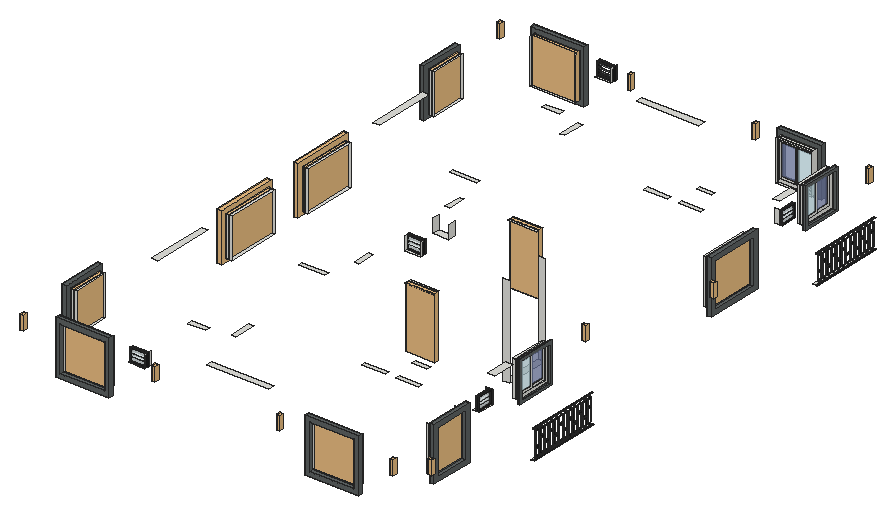
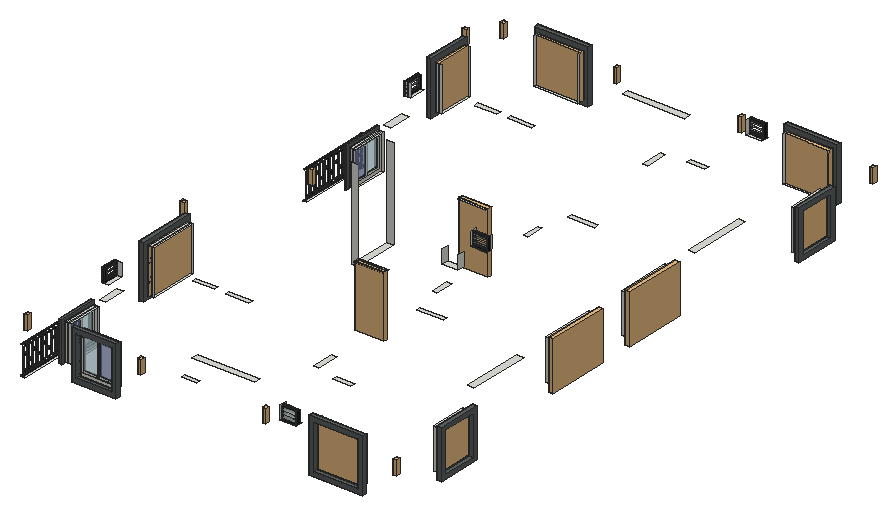
# SketchUp Ruby script. Lengths in inches.
U = 1.inch
M = Sketchup.active_model
def pt(a) = Geom::Point3d.new(a.map { |v| v * U })
def face(e, loops, mat)
  f = e.add_face(loops[0].map { |a| pt(a) })
  loops[1..].each { |l| e.add_face(l.map { |a| pt(a) }).erase! }
  f.material = f.back_material = mat if mat
  f
end
# faces: each face lists its corners as indices into pts; further lists are holes
def faces(e, pts, list, mat = nil) = list.each { |f| face(e, (f[0].is_a?(Array) ? f : [f]).map { |l| l.map { |i| pts[i] } }, mat) }
# xy, xz, yz: faces in a plane at the given z, y or x. An outline is a flat list of corners, or four numbers for a rectangle; further outlines are holes
def ring(l) = l.size == 4 ? [[l[0], l[1]], [l[2], l[1]], [l[2], l[3]], [l[0], l[3]]] : l.each_slice(2).to_a
def flat(e, list, mat, &to3) = list.each { |f| face(e, (f[0].is_a?(Array) ? f : [f]).map { |l| ring(l).map { |u, v| to3.(u, v) } }, mat) }
def xy(e, z, list, mat = nil) = flat(e, list, mat) { |x, y| [x, y, z] }
def xz(e, y, list, mat = nil) = flat(e, list, mat) { |x, z| [x, y, z] }
def yz(e, x, list, mat = nil) = flat(e, list, mat) { |y, z| [x, y, z] }
def lines(e, pts, list) = list.each { |a, b| e.add_line(pt(pts[a]), pt(pts[b])) }
# prism: a flat outline (further loops are holes) pulled along v
def prism(e, loops, v, mat = nil)
  f = face(e, loops, mat); d = Geom::Vector3d.new(v.map { |x| x * U })
  f.pushpull(f.normal.samedirection?(d) ? d.length : -d.length)
end
def box(e, o, s, mat = nil) = prism(e, [[o, [o[0] + s[0], o[1], o[2]], [o[0] + s[0], o[1] + s[1], o[2]], [o[0], o[1] + s[1], o[2]]]], [0, 0, s[2]], mat)
def at(x, y, z, deg = 0) = Geom::Transformation.translation(pt([x, y, z])) * Geom::Transformation.rotation(ORIGIN, Z_AXIS, deg.degrees)
def axes(o, x, y, z) = Geom::Transformation.new([*x, 0, *y, 0, *z, 0, *pt(o).to_a, 1])
def part(name) = M.definitions.add(name)
# library, detail: a bought-in or finely detailed component or shape, given as its bounding box
def library(name, o, s) = part(name).tap { |d| box(d.entities, o, s) }
def detail(e, o, s) = box(e.add_group.entities, o, s)
def put(e, d, t, mat = nil) = e.add_instance(d, t).tap { |i| i.material = mat if mat }
def group(e, t, mat = nil) = e.add_group.tap { |g| g.transformation = t; g.material = mat if mat }.entities
root = M.entities
M.materials.add("1487 AP 8286 CHARCOAL SHADOW").color = [94, 99, 99]
M.materials.add("[Color M08]").color = [30, 30, 30]
M.materials.add("[Color_008]1").color = [30, 30, 30]
M.materials.add("[Translucent Glass Safety]").color = [218, 227, 229]
M.materials["[Translucent Glass Safety]"].alpha = 0.5
M.materials.add("[Translucent_Glass_Safety]").color = [204, 235, 244]
M.materials["[Translucent_Glass_Safety]"].alpha = 0.5
M.materials.add("[Translucent_Glass_Sky_Reflection]").color = [125, 138, 183]
M.materials["[Translucent_Glass_Sky_Reflection]"].alpha = 0.52
c1 = library("porta 4",[0.2,-5.42,1.33],[46.55,4.72,83.21])
c2 = part("Group\#70")
prism(c2.entities,[[[4.13,0,3.9375],[7.875,0,3.9375],[7.875,0,13.78],[4.13,0,13.78],[4.13,0,15.75],[7.875,0,15.75],[7.875,0,35.43],[4.13,0,35.43],[4.13,0,39.37],[3.74,0,39.37],[3.74,0,35.43],[0,0,35.43],[0,0,15.75],[3.74,0,15.75],[3.74,0,13.78],[0,0,13.78],[0,0,3.9375],[3.74,0,3.9375],[3.74,0,0],[4.13,0,0]],[[0.39,0,16.14],[0.39,0,35.04],[7.48,0,35.04],[7.48,0,16.14]],[[7.48,0,4.33],[0.39,0,4.33],[0.39,0,13.39],[7.48,0,13.39]]],[0,0.39,0],"[Color M08]")
c3 = part("Group\#69")
prism(c3.entities,[[[3.74,0,35.43],[0,0,35.43],[0,0,25.59],[3.74,0,25.59],[3.74,0,23.62],[0,0,23.62],[0,0,3.9375],[3.74,0,3.9375],[3.74,0,0],[4.13,0,0],[4.13,0,3.9375],[7.875,0,3.9375],[7.875,0,23.62],[4.13,0,23.62],[4.13,0,25.59],[7.875,0,25.59],[7.875,0,35.43],[4.13,0,35.43],[4.13,0,39.37],[3.74,0,39.37]],[[7.48,0,23.23],[7.48,0,4.33],[0.39,0,4.33],[0.39,0,23.23]],[[0.39,0,35.04],[7.48,0,35.04],[7.48,0,25.98],[0.39,0,25.98]]],[0,0.39,0],"[Color M08]")
c4 = part("Group\#71")
put(c4.entities,c2,at(0,0,0))
put(c4.entities,c3,at(9.84,0,0))
c5 = part("Group\#79")
g1 = group(c5.entities,at(0,0,0))
box(g1,[0,-2.09,0],[1.97,122.29,0.79],"[Color M08]")
put(c5.entities,c4,axes([0.79,40.35,0.79],[0,1,0],[1,0,0],[0,0,1]))
put(c5.entities,c4,axes([0.79,79.72,0.79],[0,1,0],[1,0,0],[0,0,1]))
put(c5.entities,c4,axes([0.79,60.04,0.79],[0,1,0],[1,0,0],[0,0,1]))
put(c5.entities,c4,axes([0.79,99.41,0.79],[0,1,0],[1,0,0],[0,0,1]))
g2 = group(c5.entities,at(0,0,40.16))
box(g2,[0,-2.09,0],[1.97,122.29,0.79],"[Color M08]")
put(c5.entities,c4,axes([0.79,20.67,0.79],[0,1,0],[1,0,0],[0,0,1]))
put(c5.entities,c4,axes([0.79,0.98,0.79],[0,1,0],[1,0,0],[0,0,1]))
c6 = part("14")
prism(c6.entities,[[[0,60,66],[0,0,66],[0,0,0],[0,60,0]],[[0,54,6],[0,6,6],[0,6,60],[0,54,60]]],[-6,0,0])
c7 = library("15",[-6,0,0],[6,84,66])
c8 = part("17")
prism(c8.entities,[[[0,0,0],[0,0,72],[72,0,72],[72,0,0]],[[6,0,6],[66,0,6],[66,0,66],[6,0,66]]],[0,-6,0])
c9 = library("Group\#98",[0,-5.45,0],[91.05,108.7,8])
c10 = part("Two-panel window")
xy(c10.entities,0,[[0,0,4.33,55.51]])
xy(c10.entities,2.76,[[0,2.76,2,2.76,2,27.76,0.82,27.76,0.82,52.76,0,52.76],[3.15,2.76,4.33,2.76,4.33,52.76,2.36,52.76,2.36,27.76,3.15,27.76],[0.82,27.76,2.36,52.76]])
xy(c10.entities,4.72,[[2,4.72,2.4,26.38],[2.76,4.72,3.15,26.38],[0.82,29.13,1.22,50.79],[1.97,29.13,2.36,50.79]])
xy(c10.entities,36.61,[[2,4.72,2.4,26.38],[2.76,4.72,3.15,26.38],[0.82,29.13,1.22,50.79],[1.97,29.13,2.36,50.79]])
xy(c10.entities,38.58,[[0,2.76,2,27.76],[3.15,2.76,4.33,27.76],[0,27.76,0.82,52.76],[0.82,27.76,2.36,52.76],[2.36,27.76,4.33,52.76]])
xy(c10.entities,41.34,[[0,0,4.33,55.51]])
xz(c10.entities,0,[[0,0,4.33,41.34]])
xz(c10.entities,2.76,[[0,2.76,2,38.58],[3.15,2.76,4.33,38.58]])
xz(c10.entities,4.72,[[2,4.72,2.4,36.61],[2.76,4.72,3.15,36.61]])
xz(c10.entities,26.38,[[2,4.72,2.4,36.61],[2.76,4.72,3.15,36.61]])
xz(c10.entities,27.76,[[0.82,2.76,2,38.58],[2,2.76,2.36,38.58],[2.36,2.76,3.15,38.58]])
xz(c10.entities,29.13,[[0.82,4.72,1.22,36.61],[1.97,4.72,2.36,36.61]])
xz(c10.entities,50.79,[[0.82,4.72,1.22,36.61],[1.97,4.72,2.36,36.61]])
xz(c10.entities,52.76,[[0,2.76,0.82,38.58],[0.82,2.76,2.36,38.58],[2.36,2.76,4.33,38.58]])
xz(c10.entities,55.51,[[0,0,4.33,41.34]])
yz(c10.entities,0,[[[0,0,55.51,41.34],[2.76,2.76,52.76,38.58]]])
yz(c10.entities,0.82,[[[27.76,2.76,52.76,38.58],[29.13,4.72,50.79,36.61]]])
yz(c10.entities,1.22,[[29.13,4.72,50.79,36.61]],"[Translucent_Glass_Sky_Reflection]")
yz(c10.entities,1.97,[[29.13,4.72,50.79,36.61]],"[Translucent_Glass_Sky_Reflection]")
yz(c10.entities,2,[[[2.76,2.76,27.76,38.58],[4.72,4.72,26.38,36.61]]])
yz(c10.entities,2.36,[[[27.76,2.76,52.76,38.58],[29.13,4.72,50.79,36.61]]])
yz(c10.entities,2.4,[[4.72,4.72,26.38,36.61]],"[Translucent_Glass_Safety]")
yz(c10.entities,2.76,[[4.72,4.72,26.38,36.61]],"[Translucent_Glass_Safety]")
yz(c10.entities,3.15,[[[2.76,2.76,27.76,38.58],[4.72,4.72,26.38,36.61]]])
yz(c10.entities,4.33,[[[0,0,55.51,41.34],[2.76,2.76,52.76,38.58]]])
c11 = library("Group\#36",[0,-5.45,0],[91.05,108.7,8])
c12 = library("Group\#50",[0,-5.45,0],[91.05,108.7,8])
c13 = library("Group\#28",[0.125,0,-2.28],[4,104,84.28])
c14 = library("WALL LIGHT 69",[4.19,4.05,-9.73],[4.61,5.7,19.03])
c15 = part("Group\#40")
box(c15.entities,[0,0.25,0],[21,0.25,6],"[Translucent Glass Safety]")
c16 = part("tingkap keping toilet")
g3 = group(c16.entities,at(-23.5,-2,0),"[Color_008]1")
prism(g3,[[[47,0,57],[22.5,0,57],[22.5,0,41.8],[47,0,41.8]],[[24.5,0,43.3],[24.5,0,55.5],[45.5,0,55.5],[45.5,0,43.3]]],[0,4,0])
g4 = group(c16.entities,at(1,-2,47))
put(g4,c15,axes([0,3.73,3.53],[1,0,0],[0,0.757,0.65342],[0,-0.65342,0.757]))
put(g4,c15,axes([0,3.73,-0.17],[1,0,0],[0,0.757,0.65342],[0,-0.65342,0.757]))
put(g4,c15,axes([0,3.73,-3.87],[1,0,0],[0,0.757,0.65342],[0,-0.65342,0.757]))
xy(root,134,[[682.5,564.97,688.5,663.97],[553.5,678.97,562.5,738.97],[679.5,1044.97,685.5,1143.97]])
xy(root,162,[[649.5,897.97,658.5,963.97]])
xy(root,168,[[218,357.97,278,366.97],[554.5,357.97,614.5,366.97],[171,426.87,180,474.87],[652.5,426.87,661.5,474.87],[493.5,600.97,513.5,606.97],
  [622.5,609.97,631.5,657.97],[198,654.97,207,726.97],[198,783.97,207,855.97],[171,1029.97,180,1077.97],[493.5,1080.97,513.5,1086.97],
  [622.5,1089.97,631.5,1137.97],[218,1143.97,278,1152.97],[550.5,1143.97,598.5,1152.97]])
xy(root,210,[[306,357.97,327.5,366.97],[652.5,504.97,661.5,526.53],[382.75,726.97,404.25,735.97],[382.75,774.97,404.25,783.97],[649.5,1017.47,658.5,1038.97],
  [306,1143.97,327.5,1152.97]])
xy(root,216,[[309,453.97,333,459.97],[360,462.97,366,492.97],[507,498.97,539,504.97],[553.5,498.97,583.5,504.97],[622.5,567.97,631.5,597.97],
  [622.5,609.97,631.5,657.97],[321,624.97,357,630.97],[433.5,663.97,472.5,672.97],[363,666.97,369,690.97],[363,819.97,369,843.97],
  [433.5,837.97,472.5,846.97],[321,879.97,357,885.97],[504,978.97,536,984.97],[550.5,978.97,580.5,984.97],[360,1017.47,366,1047.47],
  [622.5,1047.97,631.5,1077.97],[309,1050.97,333,1056.97],[622.5,1089.97,631.5,1137.97]])
xy(root,222,[[386.25,387.97,470.25,396.97],[171,426.87,180,474.87],[198,530.97,207,614.97],[198,654.97,207,726.97],[198,783.97,207,855.97],
  [649.5,897.97,658.5,963.97],[198,903.97,207,987.97],[171,1029.97,180,1077.97],[386.25,1113.97,470.25,1122.97],[550.5,1143.97,598.5,1152.97]])
xz(root,426.87,[[171,168,180,222],[652.5,168,661.5,228]])
xz(root,474.87,[[171,168,180,222],[652.5,168,661.5,228]])
xz(root,526.53,[[652.5,210,661.5,228]])
xz(root,609.97,[[622.5,168,631.5,216]])
xz(root,654.97,[[198,168,207,222]])
xz(root,657.97,[[622.5,168,631.5,216]])
xz(root,678.97,[[553.5,134,562.5,258]])
xz(root,726.97,[[198,168,207,222]])
xz(root,738.97,[[553.5,134,562.5,258]])
xz(root,783.97,[[198,168,207,222]])
xz(root,855.97,[[198,168,207,222]])
xz(root,897.97,[[649.5,162,658.5,222]])
xz(root,963.97,[[649.5,162,658.5,222]])
xz(root,1017.47,[[649.5,210,658.5,228]])
xz(root,1029.97,[[171,168,180,222]])
xz(root,1077.97,[[171,168,180,222]])
xz(root,1089.97,[[622.5,168,631.5,216]])
xz(root,1137.97,[[622.5,168,631.5,216]])
yz(root,218,[[357.97,168,366.97,228],[1143.97,168,1152.97,228]])
yz(root,278,[[357.97,168,366.97,228],[1143.97,168,1152.97,228]])
yz(root,327.5,[[357.97,210,366.97,228],[1143.97,210,1152.97,228]])
yz(root,382.75,[[726.97,210,735.97,228],[774.97,210,783.97,228]])
yz(root,404.25,[[726.97,210,735.97,228],[774.97,210,783.97,228]])
yz(root,550.5,[[1143.97,168,1152.97,222]])
yz(root,554.5,[[357.97,168,366.97,228]])
yz(root,598.5,[[1143.97,168,1152.97,222]])
yz(root,614.5,[[357.97,168,366.97,228]])
put(root,c1,axes([472.67,670.54,132],[-0.83352,0,0],[0,1,0],[0,0,1]))
put(root,c1,axes([472.67,840.41,132],[-0.83352,0,0],[0,-1,0],[0,0,1]))
put(root,c5,axes([687.5,566.66,134],[-1,0,0],[0,0.80958,0],[0,0,0.9525]))
put(root,c5,axes([684.5,1046.66,134],[-1,0,0],[0,0.80958,0],[0,0,0.9525]))
g5 = group(root,at(658.5,891.97,156),"1487 AP 8286 CHARCOAL SHADOW")
prism(g5,[[[0,0,72],[0,78,72],[0,78,0],[0,0,0]],[[0,6,6],[0,72,6],[0,72,66],[0,6,66]]],[6,0,0])
put(root,c6,at(171,1023.97,162),"1487 AP 8286 CHARCOAL SHADOW")
put(root,c6,at(171,420.87,162),"1487 AP 8286 CHARCOAL SHADOW")
put(root,c7,at(198,777.97,162),"1487 AP 8286 CHARCOAL SHADOW")
put(root,c7,at(198,648.97,162),"1487 AP 8286 CHARCOAL SHADOW")
put(root,c8,at(212,357.97,162),"1487 AP 8286 CHARCOAL SHADOW")
put(root,c8,at(548.5,357.97,162),"1487 AP 8286 CHARCOAL SHADOW")
g6 = group(root,at(661.5,420.87,162),"1487 AP 8286 CHARCOAL SHADOW")
prism(g6,[[[0,0,0],[0,0,72],[0,60,72],[0,60,0]],[[0,6,66],[0,6,6],[0,54,6],[0,54,66]]],[6,0,0])
g7 = group(root,at(544.5,1152.97,162),"1487 AP 8286 CHARCOAL SHADOW")
prism(g7,[[[60,0,66],[0,0,66],[0,0,0],[60,0,0]],[[54,0,6],[6,0,6],[6,0,60],[54,0,60]]],[0,6,0])
g8 = group(root,at(212,1152.97,162),"1487 AP 8286 CHARCOAL SHADOW")
prism(g8,[[[0,0,72],[0,0,0],[72,0,0],[72,0,72]],[[66,0,66],[66,0,6],[6,0,6],[6,0,66]]],[0,6,0])
put(root,c9,axes([652.6,963.97,165.01],[0,-0.72488,0],[0,0,0.55196],[0.55,0,0]))
g9 = group(root,at(631.5,604.97,163),"1487 AP 8286 CHARCOAL SHADOW")
prism(g9,[[[0,56,2],[0,2,2],[0,2,56],[0,56,56]],[[0,53,5],[0,53,53],[0,5,53],[0,5,5]]],[3,0,0])
g10 = group(root,at(631.5,1084.97,163),"1487 AP 8286 CHARCOAL SHADOW")
prism(g10,[[[0,56,2],[0,2,2],[0,2,56],[0,56,56]],[[0,53,5],[0,53,53],[0,5,53],[0,5,5]]],[5,0,0])
put(root,c9,axes([655.6,474.87,171.01],[0,-0.52718,0],[0,0,0.55196],[0.55,0,0]))
put(root,c10,axes([625.67,609.97,168],[1,0,0],[0,0.86468,0],[0,0,1.16114]))
put(root,c10,axes([625.67,1089.97,168],[1,0,0],[0,0.86468,0],[0,0,1.16114]))
put(root,c10,axes([598.5,1147.14,168],[0,1,0],[-0.86468,0,0],[0,0,1.30629]))
put(root,c9,axes([218,363.875,171.01],[0.65898,0,0],[0,0,0.55196],[0,-0.55,0]))
put(root,c11,axes([218,1147.07,171.01],[0.65898,0,0],[0,0,0.55196],[0,0.55,0]))
put(root,c12,axes([554.5,363.875,171.01],[0.65898,0,0],[0,0,0.55196],[0,-0.55,0]))
put(root,c13,axes([198.875,654.97,169.46],[1,0,0],[0,0.69231,0],[0,0,0.64074]))
put(root,c13,axes([198.875,855.97,169.46],[1,0,0],[0,-0.69231,0],[0,0,0.64074]))
put(root,c9,axes([176.9,474.87,170.71],[0,-0.52718,0],[0,0,0.49676],[-0.55,0,0]))
put(root,c9,axes([176.9,1029.97,170.71],[0,0.52718,0],[0,0,0.49676],[-0.55,0,0]))
put(root,c14,at(642,709.2,205.375,90))
put(root,c14,at(699.24,377.55,208.64,90))
put(root,c14,at(696.49,856.8,211.25,90))
put(root,c14,at(505.9375,347.23,212.67))
put(root,c14,axes([173.78,346.73,212.67],[-1,0,0],[0,1,0],[0,0,1]))
put(root,c14,axes([350.5625,347.23,212.67],[-1,0,0],[0,1,0],[0,0,1]))
put(root,c14,at(658.9375,347.23,212.67))
put(root,c14,axes([505.9375,1163.72,212.67],[1,0,0],[0,-1,0],[0,0,1]))
put(root,c14,at(173.78,1164.22,212.67,180))
put(root,c14,at(350.5625,1163.72,212.67,180))
put(root,c14,axes([658.9375,1163.72,212.67],[1,0,0],[0,-1,0],[0,0,1]))
put(root,c16,axes([658,525.65,160.5],[0,-0.87972,0],[1,0,0],[0,0,1.18421]))
put(root,c16,axes([403.42,732.47,160.5],[-0.87972,0,0],[0,-1,0],[0,0,1.18421]))
put(root,c16,axes([658,1038.15,160.5],[0,-0.87972,0],[1,0,0],[0,0,1.18421]))
put(root,c16,axes([326.67,361.47,160.5],[-0.87972,0,0],[0,-1,0],[0,0,1.18421]))
put(root,c16,axes([326.67,1149.47,160.5],[-0.87972,0,0],[0,1,0],[0,0,1.18421]))
